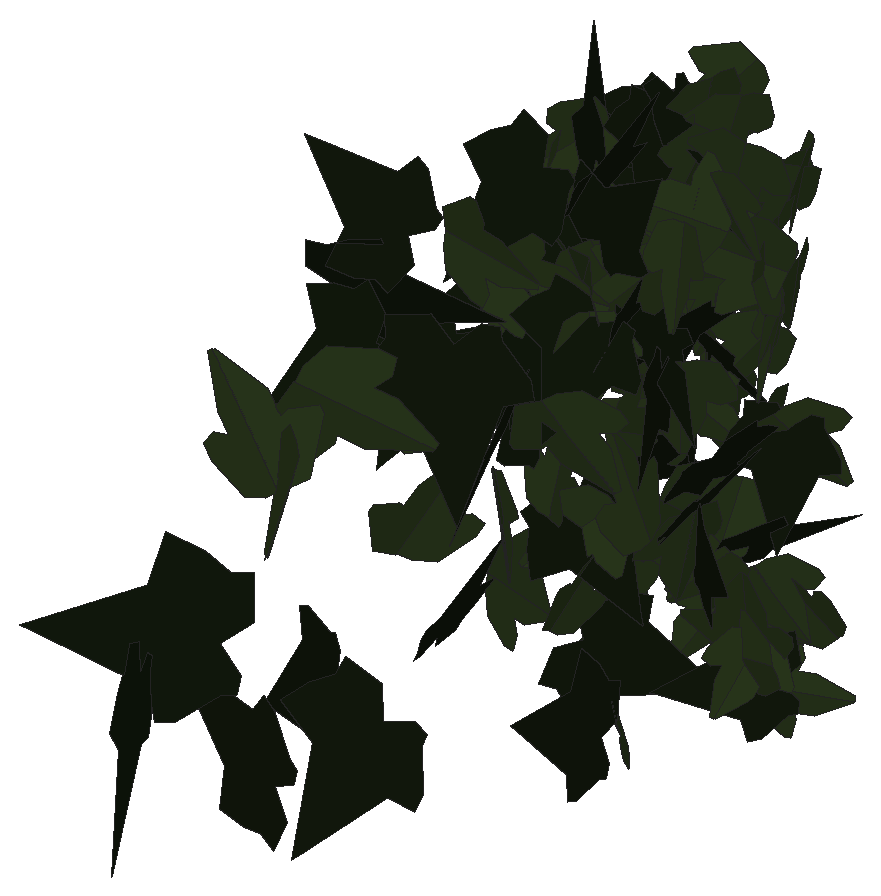
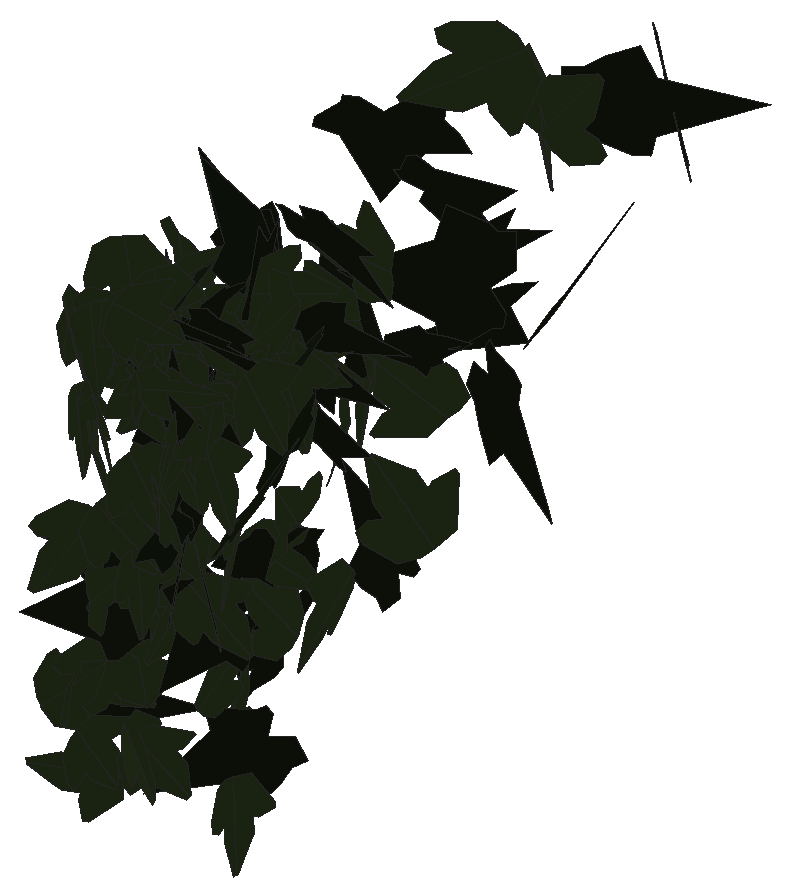
# SketchUp Ruby script. Lengths in inches.
U = 1.inch
M = Sketchup.active_model
def pt(a) = Geom::Point3d.new(a.map { |v| v * U })
def face(e, loops, mat)
  f = e.add_face(loops[0].map { |a| pt(a) })
  loops[1..].each { |l| e.add_face(l.map { |a| pt(a) }).erase! }
  f.material = f.back_material = mat if mat
  f
end
# faces: each face lists its corners as indices into pts; further lists are holes
def faces(e, pts, list, mat = nil) = list.each { |f| face(e, (f[0].is_a?(Array) ? f : [f]).map { |l| l.map { |i| pts[i] } }, mat) }
# xy, xz, yz: faces in a plane at the given z, y or x. An outline is a flat list of corners, or four numbers for a rectangle; further outlines are holes
def ring(l) = l.size == 4 ? [[l[0], l[1]], [l[2], l[1]], [l[2], l[3]], [l[0], l[3]]] : l.each_slice(2).to_a
def flat(e, list, mat, &to3) = list.each { |f| face(e, (f[0].is_a?(Array) ? f : [f]).map { |l| ring(l).map { |u, v| to3.(u, v) } }, mat) }
def xy(e, z, list, mat = nil) = flat(e, list, mat) { |x, y| [x, y, z] }
def xz(e, y, list, mat = nil) = flat(e, list, mat) { |x, z| [x, y, z] }
def yz(e, x, list, mat = nil) = flat(e, list, mat) { |y, z| [x, y, z] }
def lines(e, pts, list) = list.each { |a, b| e.add_line(pt(pts[a]), pt(pts[b])) }
# prism: a flat outline (further loops are holes) pulled along v
def prism(e, loops, v, mat = nil)
  f = face(e, loops, mat); d = Geom::Vector3d.new(v.map { |x| x * U })
  f.pushpull(f.normal.samedirection?(d) ? d.length : -d.length)
end
def box(e, o, s, mat = nil) = prism(e, [[o, [o[0] + s[0], o[1], o[2]], [o[0] + s[0], o[1] + s[1], o[2]], [o[0], o[1] + s[1], o[2]]]], [0, 0, s[2]], mat)
def at(x, y, z, deg = 0) = Geom::Transformation.translation(pt([x, y, z])) * Geom::Transformation.rotation(ORIGIN, Z_AXIS, deg.degrees)
def axes(o, x, y, z) = Geom::Transformation.new([*x, 0, *y, 0, *z, 0, *pt(o).to_a, 1])
def part(name) = M.definitions.add(name)
# library, detail: a bought-in or finely detailed component or shape, given as its bounding box
def library(name, o, s) = part(name).tap { |d| box(d.entities, o, s) }
def detail(e, o, s) = box(e.add_group.entities, o, s)
def put(e, d, t, mat = nil) = e.add_instance(d, t).tap { |i| i.material = mat if mat }
def group(e, t, mat = nil) = e.add_group.tap { |g| g.transformation = t; g.material = mat if mat }.entities
root = M.entities
M.materials.add("efeu1").color = [18, 25, 13]
M.materials.add("efeu2").color = [43, 57, 29]
c1 = part("ivyleaf_9")
p = [[1.54,2.16,1.25],[1.36,2.04,1.19],[-0.21,0.99,0.68],[-0.71,1.11,0.82],[-0.85,0.86,0.67],[-0.8,0.17,0.21],
  [-0.9,-0.01,0.1],[-0.67,-0.16,-0.02],[-0.08,-0.08,-0.05],[-0.03,-0.6,-0.4],[0.65,-0.88,-0.66],[0.83,-0.6,-0.49],
  [1.29,-0.42,-0.43],[1.8125,-0.07,-0.26],[1.21,0.44,0.15]]
faces(c1.entities,p,[[0,1,2,3,4,5,6,7,8,9,10,11,12,13,14]],"efeu1")
c2 = part("ivyleaf_10")
p = [[0,0.5,-0.03],[-0.0625,2.02,-0.43],[-0.19,2.01,-0.46],[-0.54,1.05,-0.29],[-0.52,0.625,-0.18],[-0.83,0.76,-0.28],
  [-1.16,0.64,-0.33],[-1.15,0.33,-0.24],[-0.77,-0.39,0.02],[-0.3,-0.51,0.16],[0.04,-0.48,0.23],[-0.02,2.01,-0.4375],
  [-0.06,2.01,-0.43],[0.04,-0.49,0.23],[0.67,-0.49,0.14],[1.38,0.36,-0.2],[1.375,0.51,-0.24],[0.81,0.65,-0.19],
  [0.62,0.59,-0.15],[0.6,1.09,-0.28],[0.5,1.23,-0.31]]
faces(c2.entities,p,[[0,1,2,3,4,5,6,7,8,9,10],[11,12,0,13,14,15,16,17,18,19,20]],"efeu2")
put(root,c1,axes([506.18,119.25,180.04],[-0.62449,0.18852,-0.92524],[0.92798,-0.23206,-0.63195],[-0.3217,-1.03537,-0.02683]))
put(root,c1,axes([506.31,121.0625,180.1],[-0.57418,-0.1157,0.92984],[-0.94865,-0.16724,-0.56571],[0.21924,-1.02667,-0.01264]))
put(root,c1,axes([506.05,122.98,176.47],[0.01988,-0.95853,0.23333],[0.00363,0.22445,0.99703],[-1.06319,-0.01716,0.00777]))
put(root,c2,axes([505.87,123.63,182.02],[0.55706,-0.80523,-0.30357],[-0.14501,0.2605,-0.99414],[0.91358,0.53234,0.0273]))
put(root,c1,axes([506.82,124.92,176.97],[-0.45642,-0.79531,0.34235],[-0.17953,-0.28441,-0.93656],[0.91211,-0.45396,-0.01303]))
put(root,c2,axes([504.92,124.3125,181.64],[0.84195,0.15371,0.58133],[-0.59169,-0.1109,0.82637],[0.20469,-0.95284,-0.0024]))
put(root,c2,axes([505.67,124.875,183.01],[-0.47813,-0.2224,-0.88043],[0.85781,0.29656,-0.513],[0.39722,-0.90814,0.04809]))
put(root,c1,axes([505.08,125.89,176.72],[0.0451,0.02815,-1.06352],[-1.10205,-0.07163,-0.04538],[-0.07856,1.02096,0.02614]))
put(root,c1,axes([506.28,127.59,182.81],[-0.56578,-0.65182,-0.4995],[0.35086,0.35477,-0.86925],[0.80096,-0.61584,0.02794]))
put(root,c1,axes([503.38,129.01,181.31],[-0.37683,-0.44675,0.61563],[-0.32924,-0.50996,-0.58714],[0.73014,-0.46052,0.05296]))
put(root,c1,axes([505.87,129.61,180.68],[-0.51179,0.38589,-0.62226],[0.50249,-0.37619,-0.63557],[-0.58202,-0.66411,-0.00155]))
put(root,c1,axes([503.4375,129.81,183.14],[-0.71486,-0.22748,-0.41554],[-0.39973,-0.15188,0.7276],[-0.29459,0.75809,0.02107]))
put(root,c1,axes([502.07,129.87,181.61],[0.63265,-0.03239,0.74375],[0.77047,-0.05054,-0.6101],[0.06438,0.92305,-0.00731]))
put(root,c1,axes([503.69,130.5,175.21],[0.17112,0.69597,0.30814],[-0.07529,-0.288,0.74231],[0.81345,-0.17306,0.00388]))
put(root,c2,axes([504.61,130.9375,178.0625],[-0.2867,0.55195,-0.39467],[0.17555,-0.34292,-0.63697],[-0.70179,-0.31127,0.0019]))
put(root,c1,axes([503.3,131.28,180.4],[-0.62202,-0.62265,0.05591],[-0.0415,-0.03769,-0.8821],[0.67369,-0.57722,-0.00272]))
put(root,c2,axes([502.74,130.59,179.07],[0.52451,0.31115,-0.63418],[0.56264,0.31708,0.59977],[0.47967,-0.71216,-0.01004]))
put(root,c2,axes([505.94,130.84,180.02],[-0.76121,-0.2174,-0.40012],[0.38956,0.13538,-0.7668],[0.27572,-0.7915,-0.02126]))
put(root,c2,axes([502.79,130.91,176.5625],[-0.31205,-0.73551,0.38868],[0.14472,0.3489,0.82183],[-0.87919,0.31848,-0.00267]))
put(root,c2,axes([503.45,131.35,182.24],[0.01986,-0.06328,0.82034],[0.84709,0.10604,-0.01017],[-0.11328,0.78185,0.06778]))
put(root,c2,axes([503.9,131.1,179.78],[-0.55244,0.39273,0.35056],[-0.29304,0.20008,-0.67067],[-0.47598,-0.579,0.00603]))
put(root,c1,axes([505.71,132.18,173.18],[-0.10579,-0.06323,0.8525],[-0.39409,-0.75867,-0.10517],[0.75859,-0.40295,0.06425]))
put(root,c1,axes([505.36,132.52,180.79],[-0.3552,-0.70852,0.23963],[0.03063,-0.26358,-0.80085],[0.80406,-0.30296,0.13636]))
put(root,c1,axes([504.79,132.05,180.09],[-0.35115,-0.13857,-0.67737],[-0.66083,-0.22379,0.36719],[-0.28374,0.69271,-0.01688]))
put(root,c2,axes([506.64,132.11,177.74],[-0.22103,0.84584,0.06133],[-0.0094,-0.06582,0.87387],[0.84801,0.21973,0.02567]))
put(root,c1,axes([504.18,132.5,183.4],[-0.89848,-0.07457,-0.0907],[0.09528,-0.00753,-0.86852],[0.07924,-0.83645,0.0159]))
put(root,c1,axes([504.53,132,178.75],[-0.23601,0.2354,0.64785],[-0.45736,0.45685,-0.33404],[-0.55504,-0.47654,-0.00021]))
put(root,c2,axes([504.63,132.56,180.25],[-0.05355,0.03662,0.71088],[-0.63576,-0.35204,-0.0248],[0.37729,-0.58801,0.05912]))
put(root,c2,axes([505.34,132.4375,180.66],[0.24376,0.67121,-0.14252],[-0.05759,-0.12663,-0.73639],[-0.73761,0.2317,0.0104]))
put(root,c2,axes([503.75,132.18,181.32],[0.12879,0.03031,0.84181],[0.68043,0.51073,-0.11642],[-0.5498,0.63918,0.05311]))
put(root,c1,axes([504.28,132.95,181.31],[-0.66869,-0.19453,0.46552],[-0.45926,-0.13983,-0.67493],[0.25868,-0.7511,0.00509]))
put(root,c1,axes([505.37,132.73,182.42],[-0.22963,0.1546,0.6899],[0.50223,-0.47483,0.27009],[0.53751,0.5097,0.04236]))
put(root,c2,axes([503.74,132.15,175.45],[-0.12959,0.5228,0.65635],[-0.21056,0.60131,-0.55659],[-0.85967,-0.22609,0.03739]))
put(root,c2,axes([504.57,133.12,181.05],[-0.58788,0.17378,0.47438],[0.43869,-0.21762,0.59035],[0.29234,0.67602,0.06809]))
put(root,c1,axes([503.8,133.5,180.67],[0.20992,-0.71559,0.37943],[0.11092,-0.35015,-0.77114],[0.86036,0.21974,0.00684]))
put(root,c2,axes([504.41,133.11,180.43],[-0.71728,-0.21282,0.36501],[-0.3612,-0.10642,-0.72531],[0.25698,-0.7436,-0.00066]))
put(root,c2,axes([504.76,133.35,176.54],[0.43273,0.22229,-0.58263],[-0.54878,-0.23721,-0.47584],[-0.35007,0.64663,0.02573]))
put(root,c1,axes([505.96,133.56,179.6],[-0.09121,0.08392,-0.70049],[0.60001,-0.38139,-0.12186],[-0.42114,-0.56155,-0.02192]))
put(root,c2,axes([504.45,132.94,174.78],[0.14208,-0.6265,0.40596],[-0.01945,0.39366,0.66339],[-0.79697,-0.12129,0.05618]))
put(root,c2,axes([506.5,133.34,182.42],[0.69483,-0.25039,0.19378],[0.19133,-0.05849,-0.71792],[0.27751,0.66725,0.00979]))
put(root,c2,axes([504.23,132.76,177.08],[0.0244,0.54152,-0.53597],[0.02748,0.51473,0.56367],[0.80689,-0.03391,-0.00299]))
put(root,c2,axes([505.28,133.34,172.53],[-0.53295,0.37574,0.19399],[0.14828,-0.12746,0.6448],[0.4281,0.51192,0.01816]))
put(root,c1,axes([503.66,133.78,179.1875],[0.19151,-0.54337,0.58497],[0.22129,-0.54187,-0.57578],[0.76712,0.29196,0.02006]))
put(root,c2,axes([505.61,133.65,181.4375],[-0.28766,-0.36497,0.54035],[-0.283,-0.45003,-0.46847],[0.62463,-0.37197,0.0366]))
put(root,c1,axes([505.57,132.71,180.42],[-0.20311,0.20716,-0.8038],[-0.59053,0.54547,0.2898],[0.58333,0.62434,0.01351]))
put(root,c1,axes([504.41,133.27,176.68],[0.03232,-0.54336,-0.59883],[-0.03939,0.57465,-0.56594],[0.85413,0.04706,-0.00345]))
put(root,c1,axes([504.63,133.36,182.78],[0.16291,0.73103,0.23257],[-0.08471,-0.21193,0.77555],[0.82127,-0.16687,0.03386]))
put(root,c2,axes([504.76,133.42,181.58],[-0.5014,-0.58719,-0.32247],[0.27485,0.1921,-0.77464],[0.66239,-0.52418,0.07734]))
put(root,c2,axes([505.54,133.15,178.54],[-0.17272,0.28731,0.64618],[-0.31526,0.54852,-0.34192],[-0.66872,-0.3328,-0.0057]))
put(root,c1,axes([505.23,134.12,180.39],[0.39159,-0.71506,-0.03519],[-0.03198,0.02291,-0.83364],[0.77247,0.36344,-0.01667]))
put(root,c1,axes([506.09,134.38,176.02],[0.34912,-0.31954,-0.60629],[0.69,-0.0299,0.38548],[-0.1985,-0.66593,0.27361]))
put(root,c2,axes([503.65,134.5625,183.01],[0.17205,0.19909,-0.76985],[-0.45219,-0.62341,-0.26228],[-0.65408,0.48335,-0.02118]))
put(root,c2,axes([506.05,134.21,176.45],[-0.17498,-0.72886,0.00656],[-0.0012,-0.00621,-0.77652],[0.7872,-0.16202,0.00028]))
put(root,c2,axes([506.01,134.67,182.07],[0.08047,0.45646,0.69902],[-0.18875,-0.67413,0.46193],[0.81324,-0.20163,0.03804]))
put(root,c1,axes([506.02,133.82,176.53],[-0.07889,0.64935,-0.16939],[-0.01994,0.16182,0.67958],[0.72275,0.07534,0.00026]))
put(root,c2,axes([505.38,134.22,181.34],[0.47248,0.01295,0.62457],[-0.64873,0.00496,0.45497],[0.0039,-0.74298,0.01392]))
put(root,c2,axes([505.75,134.39,179.14],[-0.66796,-0.49469,0.02485],[-0.01994,-0.01518,-0.82366],[0.53451,-0.61876,0.00033]))
put(root,c1,axes([503.92,134.36,182.85],[-0.02293,-0.40348,0.62901],[0.14862,0.59191,0.41569],[-0.77102,0.12609,0.06142]))
put(root,c2,axes([503.38,134.18,182.5],[-0.00363,0.03602,0.77467],[-0.28022,0.69828,-0.03633],[-0.75508,-0.25932,0.00976]))
put(root,c2,axes([506.11,134.93,175.52],[-0.39755,-0.24967,0.43116],[-0.35897,-0.24816,-0.46236],[0.37989,-0.49577,0.01431]))
put(root,c1,axes([505.12,135.11,180.87],[-0.01692,0.46499,0.67833],[0.00537,-0.67839,0.46517],[0.82238,0.01399,0.01092]))
put(root,c2,axes([506.72,135.08,173.91],[0.43922,0.37321,-0.31293],[-0.24806,-0.19465,-0.57396],[-0.45446,0.46695,0.01086]))
put(root,c1,axes([503.71,134.47,173.28],[0.22455,-0.07733,-0.8202],[0.11584,0.84464,-0.04792],[0.81565,-0.09867,0.23261]))
put(root,c1,axes([505.24,134.58,179.67],[0.10284,0.77674,-0.02428],[-0.00322,-0.02316,-0.81386],[-0.83925,0.09527,0.00014]))
put(root,c2,axes([507.05,134.93,173.89],[-0.14559,-0.02574,0.61088],[-0.63391,-0.02911,-0.14142],[0.03689,-0.60195,-0.01928]))
put(root,c2,axes([506.15,135.01,182.64],[-0.56072,0.17984,-0.30006],[0.28968,-0.10696,-0.5713],[-0.22563,-0.58426,0.01222]))
put(root,c1,axes([506.97,135.39,173.27],[-0.45955,-0.13644,0.5515],[-0.54247,-0.17016,-0.46469],[0.23548,-0.65827,0.00581]))
put(root,c2,axes([506.42,135.3,173.91],[-0.78903,-0.20927,0.0502],[0.06867,-0.06404,0.81244],[-0.20395,0.78803,0.07936]))
put(root,c2,axes([506.61,135.56,181.09],[-0.27744,-0.1483,-0.76142],[-0.68378,-0.33514,0.31442],[-0.36634,0.73785,-0.01023]))
put(root,c2,axes([504.07,135.54,174.54],[-0.14049,0.48935,0.50558],[0.10518,-0.49516,0.5085],[0.69571,0.17368,0.02522]))
put(root,c1,axes([506.0625,134.87,177.48],[0.06665,0.76608,0.03523],[0.01843,0.03261,-0.79917],[-0.82797,0.06239,-0.01496]))
put(root,c2,axes([506.13,135.41,176.46],[0.33758,0.6048,-0.30635],[-0.19909,-0.23538,-0.70603],[-0.69873,0.35926,0.05316]))
put(root,c2,axes([504.37,134.92,180.5625],[0.03499,0.55534,0.45097],[0.04492,0.43182,-0.57838],[-0.75962,0.05111,-0.01343]))
put(root,c1,axes([504.26,135.82,182.8],[-0.10837,-0.66942,0.18902],[-0.01127,-0.18217,-0.70378],[0.74907,-0.09959,0.01676]))
put(root,c2,axes([505,135,176.1875],[-0.15305,-0.48439,-0.58935],[0.22088,0.52944,-0.52385],[0.77425,-0.24679,0.03294]))
put(root,c2,axes([506.32,135.39,183.16],[-0.6933,-0.20216,0.22649],[-0.20998,-0.08847,-0.72174],[0.21926,-0.72397,0.02495]))
put(root,c2,axes([502.91,135.69,181.57],[-0.01606,-0.70344,0.30525],[0.03362,-0.30567,-0.70264],[0.76608,-0.00134,0.03724]))
put(root,c2,axes([504.93,135.84,182.59],[0.05496,-0.55075,0.46875],[0.13136,-0.45468,-0.54962],[0.71119,0.12655,0.06529]))
put(root,c1,axes([504.15,135.9375,182.75],[-0.74279,-0.13773,0.02069],[-0.01911,-0.01297,-0.72941],[0.14907,-0.68793,0.00961]))
put(root,c2,axes([505.05,135.41,181.2],[-0.34459,-0.44133,-0.53872],[0.36883,0.3942,-0.55885],[0.59073,-0.50356,0.03467]))
put(root,c1,axes([504.38,136.08,182.61],[-0.74444,0.01022,0.13741],[-0.14081,-0.17744,-0.69315],[0.02559,-0.67905,0.18319]))
put(root,c2,axes([503.92,136.0625,176.86],[-0.40136,-0.3555,0.47741],[-0.31042,-0.36629,-0.53373],[0.50788,-0.50482,0.05106]))
put(root,c2,axes([504.75,135.68,177.96],[-0.47642,-0.18975,-0.51841],[0.50327,0.13214,-0.51087],[0.22688,-0.69156,0.04463]))
put(root,c1,axes([506.22,135.37,175.58],[0.50477,0.07037,0.56503],[0.43317,0.44251,-0.41845],[-0.40303,0.56374,0.25793]))
put(root,c2,axes([506.52,135.96,180.09],[0.40999,-0.44449,-0.10833],[-0.06189,0.08801,-0.60775],[0.48915,0.38368,0.01391]))
put(root,c1,axes([503.84,135.47,176.36],[0.3536,0.54429,0.31701],[0.16829,0.26199,-0.66058],[-0.65239,0.36259,0.00142]))
put(root,c2,axes([504.31,136.28,179.9375],[0.04537,-0.64459,0.28294],[0.04955,-0.2799,-0.6456],[0.7022,0.0614,0.02728]))
put(root,c1,axes([504.33,136.05,183.3],[0.42851,-0.57447,-0.12397],[-0.01015,0.13766,-0.72249],[0.63356,0.39075,0.07227]))
put(root,c2,axes([503.91,136.03,181.23],[0.51123,0.47958,-0.03422],[-0.02658,-0.02167,-0.70096],[-0.48007,0.51191,0.00238]))
put(root,c1,axes([504.23,136.51,177.01],[-0.0522,-0.02203,0.75998],[0.01544,-0.76165,-0.02102],[0.76015,0.01396,0.05261]))
put(root,c2,axes([506.625,135.55,180.86],[-0.04975,0.03952,0.70628],[-0.34108,0.60163,-0.05868],[-0.65072,-0.31838,-0.02324]))
put(root,c1,axes([506.58,136.25,177.57],[-0.50881,-0.39311,-0.33451],[0.26133,0.21203,-0.63809],[0.48232,-0.52958,-0.00716]))
put(root,c2,axes([503.02,136.15,172.98],[-0.04312,-0.71516,-0.12819],[0.01856,0.12729,-0.71637],[0.72632,-0.04571,0.01069]))
put(root,c2,axes([506.25,136.04,174.71],[-0.55874,-0.3425,-0.34182],[0.32337,0.14179,-0.64382],[0.39782,-0.5963,0.04324]))
put(root,c2,axes([506.51,136.45,182.26],[-0.10482,-0.62984,0.28599],[-0.031,-0.28469,-0.63833],[0.69104,-0.10831,0.01475]))
put(root,c1,axes([502.6,136.74,179.09],[0.35802,-0.64465,-0.23053],[0.10789,-0.20377,0.73738],[-0.67607,-0.3739,-0.0044]))
put(root,c2,axes([504.84,136.58,173.54],[-0.34561,-0.38296,0.42339],[-0.15938,-0.41053,-0.50143],[0.5482,-0.36079,0.12115]))
put(root,c2,axes([504.75,136.34,183.44],[-0.2025,-0.66459,-0.02454],[0.01088,0.02167,-0.71814],[0.71813,-0.18773,0.00396]))
put(root,c2,axes([506,136.6,179.55],[0.55166,-0.48064,0.25433],[0.18126,-0.17904,-0.73152],[0.51269,0.58048,-0.01503]))
put(root,c1,axes([503.4,136.67,177.8125],[-0.37865,0.06007,-0.67401],[0.655,-0.16141,-0.38236],[-0.16992,-0.75605,0.02808]))
put(root,c2,axes([504.87,136.45,181.28],[0.53209,0.42814,-0.22657],[-0.26845,-0.03985,-0.66603],[-0.44396,0.53722,0.13117]))
put(root,c1,axes([504.43,136.28,178.72],[0.77082,-0.16365,0.08586],[0.08389,-0.0183,-0.788],[0.16467,0.77537,-0.00048]))
put(root,c2,axes([504.23,136.13,180.68],[0.07827,-0.57667,-0.49339],[0.08912,0.49955,-0.56974],[0.75368,0.00082,0.11861]))
put(root,c2,axes([503.17,136.64,180.28],[0.03484,-0.6922,0.12796],[0.02231,-0.12697,-0.6929],[0.70358,0.0383,0.01563]))
put(root,c2,axes([507.0625,136.52,173.9],[-0.4796,0.07582,-0.47593],[-0.49513,0.02476,0.46694],[0.07631,0.63719,0.03848]))
put(root,c2,axes([506.07,136.35,172.48],[-0.03282,-0.00615,-0.71925],[0.74151,0.08311,-0.03215],[0.08996,-0.68725,0.00255]))
put(root,c2,axes([506.17,136.52,182.29],[-0.16403,-0.67863,-0.0397],[-0.00464,0.04195,-0.69802],[0.67977,-0.16347,-0.01434]))
put(root,c2,axes([502.92,136.3125,178.625],[-0.42503,0.51446,0.15576],[-0.11912,0.10349,-0.66685],[-0.52416,-0.44069,0.02524]))
put(root,c2,axes([504.92,136.72,182.88],[-0.18515,-0.64663,0.20315],[-0.05462,-0.19567,-0.67261],[0.67559,-0.19304,0.0013]))
put(root,c2,axes([504.9,136.76,179.63],[-0.32856,-0.58881,0.2804],[-0.09044,-0.26981,-0.67254],[0.64587,-0.33732,0.04847]))
put(root,c2,axes([506.52,136.33,177.625],[-0.55567,-0.30294,-0.44533],[0.38794,0.21874,-0.63287],[0.37362,-0.67767,-0.0052]))
put(root,c1,axes([504.98,136.22,180.82],[-0.16584,0.18295,0.73012],[-0.44289,0.58079,-0.24613],[-0.6086,-0.47251,-0.01984]))
put(root,c2,axes([505.11,136.66,183.08],[-0.34103,-0.60164,0.13266],[-0.05091,-0.12359,-0.69138],[0.61399,-0.34442,0.01635]))
put(root,c2,axes([506.42,136.6,180.49],[0.15212,-0.65836,-0.1441],[-0.0107,0.14535,-0.67536],[0.67386,0.15093,0.02181]))
put(root,c2,axes([504.73,136.52,182.01],[-0.17725,0.70809,0.03896],[-0.00668,0.03848,-0.72993],[-0.70913,-0.17735,-0.00286]))
put(root,c2,axes([505.93,137.02,173.51],[-0.14484,-0.54371,0.37865],[0.0591,-0.39665,-0.54694],[0.65993,-0.08381,0.13209]))
put(root,c2,axes([504.42,136.84,181.52],[0.02238,0.33325,0.63084],[-0.6018,-0.3302,0.19579],[0.38323,-0.53799,0.2706]))
put(root,c2,axes([506.45,136.84,182.53],[0.36153,-0.57677,0.0556],[0.05327,-0.03314,-0.69303],[0.62331,0.33737,0.02698]))
put(root,c2,axes([504.86,136.74,177.58],[-0.09337,-0.67371,-0.07354],[0.0188,0.07163,-0.6801],[0.67745,-0.09484,0.00874]))
put(root,c2,axes([504.86,136.94,173.91],[0.2125,-0.65227,0.15038],[0.03845,-0.14562,-0.68596],[0.66828,0.21579,-0.00836]))
put(root,c2,axes([505.48,137.3,177],[-0.06587,0.04333,-0.70255],[-0.02322,-0.70537,-0.04133],[-0.70351,0.01923,0.06715]))
put(root,c2,axes([505.32,137.1,178.59],[-0.30959,-0.43686,0.45969],[-0.24255,-0.39108,-0.535],[0.58594,-0.39271,0.02142]))
put(root,c2,axes([503.25,136.71,181.16],[-0.07374,0.69346,0.04447],[-0.10137,0.03351,-0.69058],[-0.68745,-0.07932,0.09706]))
put(root,c2,axes([504.69,137.29,183.36],[-0.2242,-0.35256,0.57167],[-0.10697,-0.57624,-0.39733],[0.66307,-0.21217,0.1292]))
put(root,c2,axes([504.05,137.05,179.23],[0.51214,-0.28134,0.36102],[0.33461,-0.13951,-0.58339],[0.31229,0.61087,0.03303]))
